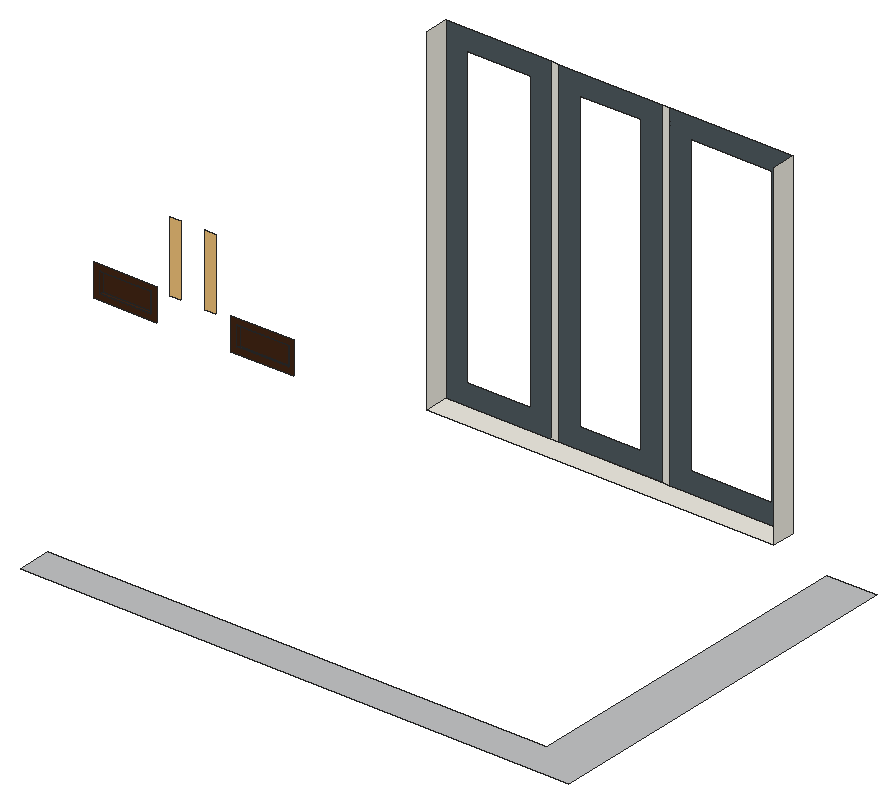
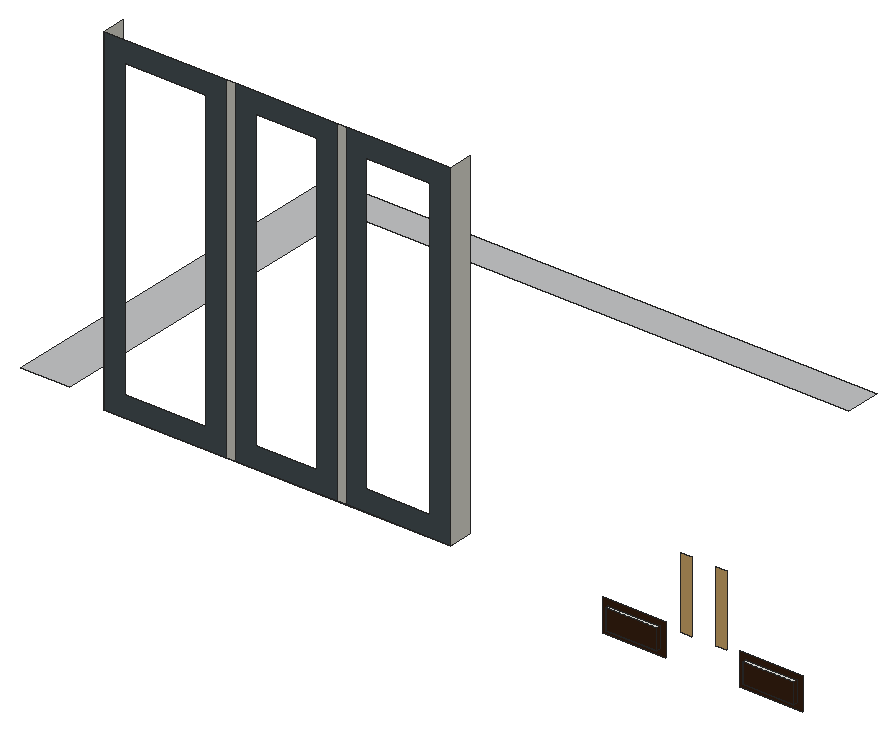
# SketchUp Ruby script. Lengths in inches.
U = 1.inch
M = Sketchup.active_model
def pt(a) = Geom::Point3d.new(a.map { |v| v * U })
def face(e, loops, mat)
  f = e.add_face(loops[0].map { |a| pt(a) })
  loops[1..].each { |l| e.add_face(l.map { |a| pt(a) }).erase! }
  f.material = f.back_material = mat if mat
  f
end
# faces: each face lists its corners as indices into pts; further lists are holes
def faces(e, pts, list, mat = nil) = list.each { |f| face(e, (f[0].is_a?(Array) ? f : [f]).map { |l| l.map { |i| pts[i] } }, mat) }
# xy, xz, yz: faces in a plane at the given z, y or x. An outline is a flat list of corners, or four numbers for a rectangle; further outlines are holes
def ring(l) = l.size == 4 ? [[l[0], l[1]], [l[2], l[1]], [l[2], l[3]], [l[0], l[3]]] : l.each_slice(2).to_a
def flat(e, list, mat, &to3) = list.each { |f| face(e, (f[0].is_a?(Array) ? f : [f]).map { |l| ring(l).map { |u, v| to3.(u, v) } }, mat) }
def xy(e, z, list, mat = nil) = flat(e, list, mat) { |x, y| [x, y, z] }
def xz(e, y, list, mat = nil) = flat(e, list, mat) { |x, z| [x, y, z] }
def yz(e, x, list, mat = nil) = flat(e, list, mat) { |y, z| [x, y, z] }
def lines(e, pts, list) = list.each { |a, b| e.add_line(pt(pts[a]), pt(pts[b])) }
# prism: a flat outline (further loops are holes) pulled along v
def prism(e, loops, v, mat = nil)
  f = face(e, loops, mat); d = Geom::Vector3d.new(v.map { |x| x * U })
  f.pushpull(f.normal.samedirection?(d) ? d.length : -d.length)
end
def box(e, o, s, mat = nil) = prism(e, [[o, [o[0] + s[0], o[1], o[2]], [o[0] + s[0], o[1] + s[1], o[2]], [o[0], o[1] + s[1], o[2]]]], [0, 0, s[2]], mat)
def at(x, y, z, deg = 0) = Geom::Transformation.translation(pt([x, y, z])) * Geom::Transformation.rotation(ORIGIN, Z_AXIS, deg.degrees)
def axes(o, x, y, z) = Geom::Transformation.new([*x, 0, *y, 0, *z, 0, *pt(o).to_a, 1])
def part(name) = M.definitions.add(name)
# library, detail: a bought-in or finely detailed component or shape, given as its bounding box
def library(name, o, s) = part(name).tap { |d| box(d.entities, o, s) }
def detail(e, o, s) = box(e.add_group.entities, o, s)
def put(e, d, t, mat = nil) = e.add_instance(d, t).tap { |i| i.material = mat if mat }
def group(e, t, mat = nil) = e.add_group.tap { |g| g.transformation = t; g.material = mat if mat }.entities
root = M.entities
M.materials.add("[Fencing Metal Straight]").color = [194, 195, 196]
M.materials.add("[Formica Speckled Grey]").color = [79, 89, 94]
M.materials.add("[Tile Limestone Large]").color = [237, 234, 224]
M.materials.add("[Wood OSB]").color = [240, 195, 122]
M.materials.add("[Wood Veneer 01]").color = [66, 38, 20]
xy(root,106.04,[[208.9,244.48,240.1,246.61],[292.21,244.48,323.42,246.42]],"[Wood Veneer 01]")
xy(root,115.1875,[[356.09,0,689.3,0,689.3,233.86,659.08,233.86,659.08,21.02,356.09,21.02]],"[Fencing Metal Straight]")
xy(root,118.43,[[208.9,244.48,240.1,246.61],[292.21,244.48,323.42,246.42]])
xy(root,120.45,[[416.36,233.86,627.05,248.23]],"[Tile Limestone Large]")
xz(root,244.48,[[251.23,119.67,257.85,162.8],[272.6,119.67,279.23,162.8]],"[Wood OSB]")
xz(root,244.48,[[[205.34,102.49,243.66,121.99],[208.9,106.04,240.1,118.43]],[[288.66,102.49,326.97,121.99],[292.21,106.04,323.42,118.43]]],"[Wood Veneer 01]")
xz(root,246.42,[[292.21,106.04,323.42,118.43]],"[Wood Veneer 01]")
xz(root,246.61,[[208.9,106.04,240.1,118.43]],"[Wood Veneer 01]")
xz(root,248.23,[[[416.36,120.45,480.22,326.11],[428.85,132.9375,467.73,313.62]],[[485.03,120.45,547.17,326.11],[497.52,132.9375,534.68,313.62]],[[552.31,120.45,627.05,326.11],[564.8,132.9375,614.56,313.62]]],"[Formica Speckled Grey]")
xz(root,248.23,[[480.22,120.45,485.03,326.11],[547.17,120.45,552.31,326.11]],"[Tile Limestone Large]")
yz(root,208.9,[[244.48,106.04,246.61,118.43]],"[Wood Veneer 01]")
yz(root,240.1,[[244.48,106.04,246.61,118.43]],"[Wood Veneer 01]")
yz(root,292.21,[[244.48,106.04,246.42,118.43]],"[Wood Veneer 01]")
yz(root,323.42,[[244.48,106.04,246.42,118.43]],"[Wood Veneer 01]")
yz(root,416.36,[[233.86,120.45,248.23,326.11]],"[Tile Limestone Large]")
yz(root,627.05,[[233.86,120.45,248.23,326.11]],"[Tile Limestone Large]")
